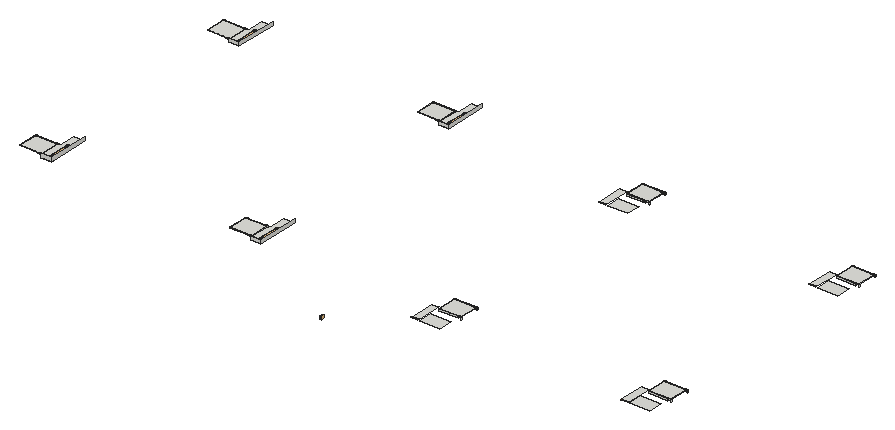
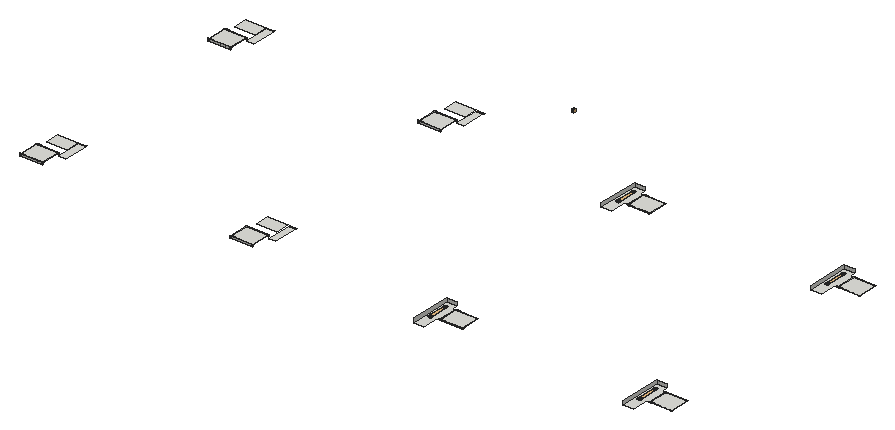
# SketchUp Ruby script. Lengths in inches.
U = 1.inch
M = Sketchup.active_model
def pt(a) = Geom::Point3d.new(a.map { |v| v * U })
def face(e, loops, mat)
  f = e.add_face(loops[0].map { |a| pt(a) })
  loops[1..].each { |l| e.add_face(l.map { |a| pt(a) }).erase! }
  f.material = f.back_material = mat if mat
  f
end
# faces: each face lists its corners as indices into pts; further lists are holes
def faces(e, pts, list, mat = nil) = list.each { |f| face(e, (f[0].is_a?(Array) ? f : [f]).map { |l| l.map { |i| pts[i] } }, mat) }
# xy, xz, yz: faces in a plane at the given z, y or x. An outline is a flat list of corners, or four numbers for a rectangle; further outlines are holes
def ring(l) = l.size == 4 ? [[l[0], l[1]], [l[2], l[1]], [l[2], l[3]], [l[0], l[3]]] : l.each_slice(2).to_a
def flat(e, list, mat, &to3) = list.each { |f| face(e, (f[0].is_a?(Array) ? f : [f]).map { |l| ring(l).map { |u, v| to3.(u, v) } }, mat) }
def xy(e, z, list, mat = nil) = flat(e, list, mat) { |x, y| [x, y, z] }
def xz(e, y, list, mat = nil) = flat(e, list, mat) { |x, z| [x, y, z] }
def yz(e, x, list, mat = nil) = flat(e, list, mat) { |y, z| [x, y, z] }
def lines(e, pts, list) = list.each { |a, b| e.add_line(pt(pts[a]), pt(pts[b])) }
# prism: a flat outline (further loops are holes) pulled along v
def prism(e, loops, v, mat = nil)
  f = face(e, loops, mat); d = Geom::Vector3d.new(v.map { |x| x * U })
  f.pushpull(f.normal.samedirection?(d) ? d.length : -d.length)
end
def box(e, o, s, mat = nil) = prism(e, [[o, [o[0] + s[0], o[1], o[2]], [o[0] + s[0], o[1] + s[1], o[2]], [o[0], o[1] + s[1], o[2]]]], [0, 0, s[2]], mat)
def at(x, y, z, deg = 0) = Geom::Transformation.translation(pt([x, y, z])) * Geom::Transformation.rotation(ORIGIN, Z_AXIS, deg.degrees)
def axes(o, x, y, z) = Geom::Transformation.new([*x, 0, *y, 0, *z, 0, *pt(o).to_a, 1])
def part(name) = M.definitions.add(name)
# library, detail: a bought-in or finely detailed component or shape, given as its bounding box
def library(name, o, s) = part(name).tap { |d| box(d.entities, o, s) }
def detail(e, o, s) = box(e.add_group.entities, o, s)
def put(e, d, t, mat = nil) = e.add_instance(d, t).tap { |i| i.material = mat if mat }
def group(e, t, mat = nil) = e.add_group.tap { |g| g.transformation = t; g.material = mat if mat }.entities
root = M.entities
M.materials.add("[Wood Veneer 01]").color = [76, 44, 23]
c1 = library("Spot Light",[-5.1,-5.1,-11.05],[10.2,10.2,11.05])
c2 = library("Group\#22",[-0.5,-0.5,-0.1],[13.19,93.55,0.2])
xy(root,93.875,[[2442.07,929.16,2442.76,929.47],[3334.66,929.16,3335.34,929.47],[2442.07,1928.52,2442.76,1928.83],[3334.66,1928.52,3335.34,1928.83]])
xy(root,97,[[563.18,847.15,656.89,931.09],[656.89,847.15,657.58,930.4],[1455.77,847.15,1549.48,931.09],[1549.48,847.15,1550.17,930.4],[563.18,931.09,645.68,931.22],
  [645.68,931.09,656.89,931.22],[1455.77,931.09,1538.27,931.22],[1538.27,931.09,1549.48,931.22],[563.18,1846.51,656.89,1930.45],[656.89,1846.51,657.58,1929.76],
  [1455.77,1846.51,1549.48,1930.45],[1549.48,1846.51,1550.17,1929.76],[563.18,1930.45,645.68,1930.57],[645.68,1930.45,656.89,1930.57],[1455.77,1930.45,1538.27,1930.57],
  [1538.27,1930.45,1549.48,1930.57]])
xy(root,97.25,[[656.89,847.15,657.58,930.4],[657.58,847.15,658.26,931.09],[1549.48,847.15,1550.17,930.4],[1550.17,847.15,1550.85,931.09],[656.89,930.4,657.58,931.09],
  [1549.48,930.4,1550.17,931.09],[656.89,931.09,657.58,931.47],[657.58,931.09,658.26,931.22],[1549.48,931.09,1550.17,931.47],[1550.17,931.09,1550.85,931.22],
  [656.89,1846.51,657.58,1929.76],[657.58,1846.51,658.26,1930.45],[1549.48,1846.51,1550.17,1929.76],[1550.17,1846.51,1550.85,1930.45],[656.89,1929.76,657.58,1930.45],
  [1549.48,1929.76,1550.17,1930.45],[656.89,1930.45,657.58,1930.82],[657.58,1930.45,658.26,1930.57],[1549.48,1930.45,1550.17,1930.82],[1550.17,1930.45,1550.85,1930.57]])
xy(root,97.9375,[[[671.36,824.85,671.36,847.15,662.14,847.15,662.14,931.78,671.36,931.78,671.36,1001.66,715.11,1001.66,715.11,824.85],[696.3,929.17,697.88,929.375,699.35,929.98,700.61,930.95,701.58,932.21,702.1875,933.68,702.39,935.26,702.1875,936.84,701.58,938.31,700.61,939.57,699.35,940.54,697.88,941.14,696.3,941.35,694.73,941.14,693.26,940.54,691.99,939.57,691.03,938.31,690.42,936.84,690.21,935.26,690.42,933.68,691.03,932.21,691.99,930.95,693.26,929.98,694.73,929.375],[696.3,848.8,697.85,849.01,699.3,849.6,700.54,850.56,701.5,851.8,702.1,853.25,702.3,854.8,702.1,856.35,701.5,857.8,700.54,859.04,699.3,860,697.85,860.6,696.3,860.8,694.75,860.6,693.3,860,692.06,859.04,691.11,857.8,690.51,856.35,690.3,854.8,690.51,853.25,691.11,851.8,692.06,850.56,693.3,849.6,694.75,849.01]],[[1563.95,824.85,1563.95,847.15,1554.73,847.15,1554.73,931.78,1563.95,931.78,1563.95,1001.66,1607.7,1001.66,1607.7,824.85],[1588.89,929.17,1590.47,929.375,1591.9375,929.98,1593.2,930.95,1594.17,932.21,1594.78,933.68,1594.98,935.26,1594.78,936.84,1594.17,938.31,1593.2,939.57,1591.9375,940.54,1590.47,941.14,1588.89,941.35,1587.31,941.14,1585.85,940.54,1584.58,939.57,1583.62,938.31,1583.01,936.84,1582.8,935.26,1583.01,933.68,1583.62,932.21,1584.58,930.95,1585.85,929.98,1587.31,929.375],[1588.89,848.8,1590.44,849.01,1591.89,849.6,1593.13,850.56,1594.09,851.8,1594.6875,853.25,1594.89,854.8,1594.6875,856.35,1594.09,857.8,1593.13,859.04,1591.89,860,1590.44,860.6,1588.89,860.8,1587.34,860.6,1585.89,860,1584.65,859.04,1583.7,857.8,1583.1,856.35,1582.89,854.8,1583.1,853.25,1583.7,851.8,1584.65,850.56,1585.89,849.6,1587.34,849.01]],[563.18,847.15,656.89,931.09],[656.89,847.15,657.58,931.78],[1455.77,847.15,1549.48,931.09],
  [1549.48,847.15,1550.17,931.78],[563.18,931.09,656.89,931.78],[657.58,931.09,658.26,931.09,658.26,931.22,662.14,931.22,662.14,931.78,657.58,931.78],[658.26,931.09,662.14,931.22],[1455.77,931.09,1549.48,931.78],
  [1550.17,931.09,1550.85,931.09,1550.85,931.22,1554.73,931.22,1554.73,931.78,1550.17,931.78],[1550.85,931.09,1554.73,931.22],[[671.36,1824.2,671.36,1846.51,662.14,1846.51,662.14,1931.13,671.36,1931.13,671.36,2001.02,715.11,2001.02,715.11,1824.2],[696.3,1928.52,697.88,1928.73,699.35,1929.34,700.61,1930.31,701.58,1931.57,702.1875,1933.04,702.39,1934.61,702.1875,1936.19,701.58,1937.66,700.61,1938.92,699.35,1939.89,697.88,1940.5,696.3,1940.71,694.73,1940.5,693.26,1939.89,691.99,1938.92,691.03,1937.66,690.42,1936.19,690.21,1934.61,690.42,1933.04,691.03,1931.57,691.99,1930.31,693.26,1929.34,694.73,1928.73],[696.3,1848.16,697.85,1848.36,699.3,1848.96,700.54,1849.91,701.5,1851.16,702.1,1852.6,702.3,1854.16,702.1,1855.71,701.5,1857.16,700.54,1858.4,699.3,1859.35,697.85,1859.95,696.3,1860.16,694.75,1859.95,693.3,1859.35,692.06,1858.4,691.11,1857.16,690.51,1855.71,690.3,1854.16,690.51,1852.6,691.11,1851.16,692.06,1849.91,693.3,1848.96,694.75,1848.36]],[[1563.95,1824.2,1563.95,1846.51,1554.73,1846.51,1554.73,1931.13,1563.95,1931.13,1563.95,2001.02,1607.7,2001.02,1607.7,1824.2],[1588.89,1928.52,1590.47,1928.73,1591.9375,1929.34,1593.2,1930.31,1594.17,1931.57,1594.78,1933.04,1594.98,1934.61,1594.78,1936.19,1594.17,1937.66,1593.2,1938.92,1591.9375,1939.89,1590.47,1940.5,1588.89,1940.71,1587.31,1940.5,1585.85,1939.89,1584.58,1938.92,1583.62,1937.66,1583.01,1936.19,1582.8,1934.61,1583.01,1933.04,1583.62,1931.57,1584.58,1930.31,1585.85,1929.34,1587.31,1928.73],[1588.89,1848.16,1590.44,1848.36,1591.89,1848.96,1593.13,1849.91,1594.09,1851.16,1594.6875,1852.6,1594.89,1854.16,1594.6875,1855.71,1594.09,1857.16,1593.13,1858.4,1591.89,1859.35,1590.44,1859.95,1588.89,1860.16,1587.34,1859.95,1585.89,1859.35,1584.65,1858.4,1583.7,1857.16,1583.1,1855.71,1582.89,1854.16,1583.1,1852.6,1583.7,1851.16,1584.65,1849.91,1585.89,1848.96,1587.34,1848.36]],[563.18,1846.51,656.89,1930.45],
  [656.89,1846.51,657.58,1931.13],[1455.77,1846.51,1549.48,1930.45],[1549.48,1846.51,1550.17,1931.13],[563.18,1930.45,656.89,1931.13],[657.58,1930.45,658.26,1930.45,658.26,1930.57,662.14,1930.57,662.14,1931.13,657.58,1931.13],
  [658.26,1930.45,662.14,1930.57],[1455.77,1930.45,1549.48,1931.13],[1550.17,1930.45,1550.85,1930.45,1550.85,1930.57,1554.73,1930.57,1554.73,1931.13,1550.17,1931.13],[1550.85,1930.45,1554.73,1930.57]])
xy(root,97.96,[[2346.59,747.5625,2430.86,806.0625],[3239.18,747.5625,3323.45,806.0625],[2346.59,1746.92,2430.86,1805.42],[3239.18,1746.92,3323.45,1805.42]])
xy(root,97.99,[[2308.36,747.5625,2338.14,753.47],[3200.95,747.5625,3230.73,753.47],[2308.36,1746.92,2338.14,1752.82],[3200.95,1746.92,3230.73,1752.82]],"[Wood Veneer 01]")
xy(root,101.6875,[[2348.36,844.85,2442.07,928.79],[2442.07,844.85,2442.76,928.1],[3240.94,844.85,3334.66,928.79],[3334.66,844.85,3335.34,928.1],[2348.36,928.79,2430.86,928.91],
  [2430.86,928.79,2442.07,928.91],[3240.94,928.79,3323.45,928.91],[3323.45,928.79,3334.66,928.91],[2348.36,1844.2,2442.07,1928.14],[2442.07,1844.2,2442.76,1927.45],
  [3240.94,1844.2,3334.66,1928.14],[3334.66,1844.2,3335.34,1927.45],[2348.36,1928.14,2430.86,1928.27],[2430.86,1928.14,2442.07,1928.27],[3240.94,1928.14,3323.45,1928.27],
  [3323.45,1928.14,3334.66,1928.27]])
xy(root,101.9375,[[2442.07,844.85,2442.76,928.1],[2442.76,844.85,2443.44,928.79],[3334.66,844.85,3335.34,928.1],[3335.34,844.85,3336.03,928.79],[2442.07,928.1,2442.76,928.79],
  [3334.66,928.1,3335.34,928.79],[2442.07,928.79,2442.76,929.16],[2442.76,928.79,2443.44,928.91],[3334.66,928.79,3335.34,929.16],[3335.34,928.79,3336.03,928.91],
  [2442.07,1844.2,2442.76,1927.45],[2442.76,1844.2,2443.44,1928.14],[3334.66,1844.2,3335.34,1927.45],[3335.34,1844.2,3336.03,1928.14],[2442.07,1927.45,2442.76,1928.14],
  [3334.66,1927.45,3335.34,1928.14],[2442.07,1928.14,2442.76,1928.52],[2442.76,1928.14,2443.44,1928.27],[3334.66,1928.14,3335.34,1928.52],[3335.34,1928.14,3336.03,1928.27]])
xz(root,824.85,[[671.36,97.9375,715.11,113.8125],[1563.95,97.9375,1607.7,113.8125]])
xz(root,844.85,[[2348.36,93.875,2430.86,101.6875],[2442.07,93.875,2442.76,101.6875],[2442.76,93.875,2447.32,93.875,2447.32,102.625,2443.44,102.625,2443.44,101.9375,2442.76,101.9375],[3240.94,93.875,3323.45,101.6875],[3334.66,93.875,3335.34,101.6875],
  [3335.34,93.875,3339.91,93.875,3339.91,102.625,3336.03,102.625,3336.03,101.9375,3335.34,101.9375],[2348.36,101.6875,2430.86,101.9375],[2430.86,101.6875,2442.07,101.9375],[2442.07,101.6875,2442.76,101.9375],[3240.94,101.6875,3323.45,101.9375],
  [3323.45,101.6875,3334.66,101.9375],[3334.66,101.6875,3335.34,101.9375],[2348.36,101.9375,2442.07,102.625],[2442.07,101.9375,2442.76,102.625],[2442.76,101.9375,2443.44,102.625],
  [3240.94,101.9375,3334.66,102.625],[3334.66,101.9375,3335.34,102.625],[3335.34,101.9375,3336.03,102.625]])
xz(root,847.15,[[563.18,97,645.68,97.25],[645.68,97,656.89,97.25],[656.89,97,657.58,97.25],[1455.77,97,1538.27,97.25],[1538.27,97,1549.48,97.25],
  [1549.48,97,1550.17,97.25],[563.18,97.25,656.89,97.9375],[656.89,97.25,657.58,97.9375],[657.58,97.25,658.26,97.9375],[1455.77,97.25,1549.48,97.9375],
  [1549.48,97.25,1550.17,97.9375],[1550.17,97.25,1550.85,97.9375]])
xz(root,928.1,[[2442.07,101.6875,2442.76,101.9375],[3334.66,101.6875,3335.34,101.9375]])
xz(root,928.79,[[2348.36,101.6875,2430.86,101.9375],[2430.86,101.6875,2442.07,101.9375],[3240.94,101.6875,3323.45,101.9375],[3323.45,101.6875,3334.66,101.9375],[2348.36,101.9375,2442.07,102.625],
  [2442.76,101.9375,2443.44,102.625],[3240.94,101.9375,3334.66,102.625],[3335.34,101.9375,3336.03,102.625]])
xz(root,929.16,[[2442.07,93.875,2442.76,101.9375],[3334.66,93.875,3335.34,101.9375]])
xz(root,929.47,[[2348.36,93.875,2442.07,102.625],[2442.07,93.875,2442.76,102.625],[2442.76,93.875,2447.32,102.625],[3240.94,93.875,3334.66,102.625],[3334.66,93.875,3335.34,102.625],
  [3335.34,93.875,3339.91,102.625]])
xz(root,930.4,[[656.89,97,657.58,97.25],[1549.48,97,1550.17,97.25]])
xz(root,931.09,[[563.18,97,645.68,97.25],[645.68,97,656.89,97.25],[1455.77,97,1538.27,97.25],[1538.27,97,1549.48,97.25],[563.18,97.25,656.89,97.9375],
  [657.58,97.25,658.26,97.9375],[1455.77,97.25,1549.48,97.9375],[1550.17,97.25,1550.85,97.9375]])
xz(root,1824.2,[[671.36,97.9375,715.11,113.8125],[1563.95,97.9375,1607.7,113.8125]])
xz(root,1844.2,[[2348.36,93.875,2430.86,101.6875],[2442.07,93.875,2442.76,101.6875],[2442.76,93.875,2447.32,93.875,2447.32,102.625,2443.44,102.625,2443.44,101.9375,2442.76,101.9375],[3240.94,93.875,3323.45,101.6875],[3334.66,93.875,3335.34,101.6875],
  [3335.34,93.875,3339.91,93.875,3339.91,102.625,3336.03,102.625,3336.03,101.9375,3335.34,101.9375],[2348.36,101.6875,2430.86,101.9375],[2430.86,101.6875,2442.07,101.9375],[2442.07,101.6875,2442.76,101.9375],[3240.94,101.6875,3323.45,101.9375],
  [3323.45,101.6875,3334.66,101.9375],[3334.66,101.6875,3335.34,101.9375],[2348.36,101.9375,2442.07,102.625],[2442.07,101.9375,2442.76,102.625],[2442.76,101.9375,2443.44,102.625],
  [3240.94,101.9375,3334.66,102.625],[3334.66,101.9375,3335.34,102.625],[3335.34,101.9375,3336.03,102.625]])
xz(root,1846.51,[[563.18,97,645.68,97.25],[645.68,97,656.89,97.25],[656.89,97,657.58,97.25],[1455.77,97,1538.27,97.25],[1538.27,97,1549.48,97.25],
  [1549.48,97,1550.17,97.25],[563.18,97.25,656.89,97.9375],[656.89,97.25,657.58,97.9375],[657.58,97.25,658.26,97.9375],[1455.77,97.25,1549.48,97.9375],
  [1549.48,97.25,1550.17,97.9375],[1550.17,97.25,1550.85,97.9375]])
xz(root,1927.45,[[2442.07,101.6875,2442.76,101.9375],[3334.66,101.6875,3335.34,101.9375]])
xz(root,1928.14,[[2348.36,101.6875,2430.86,101.9375],[2430.86,101.6875,2442.07,101.9375],[3240.94,101.6875,3323.45,101.9375],[3323.45,101.6875,3334.66,101.9375],[2348.36,101.9375,2442.07,102.625],
  [2442.76,101.9375,2443.44,102.625],[3240.94,101.9375,3334.66,102.625],[3335.34,101.9375,3336.03,102.625]])
xz(root,1928.52,[[2442.07,93.875,2442.76,101.9375],[3334.66,93.875,3335.34,101.9375]])
xz(root,1928.83,[[2348.36,93.875,2442.07,102.625],[2442.07,93.875,2442.76,102.625],[2442.76,93.875,2447.32,102.625],[3240.94,93.875,3334.66,102.625],[3334.66,93.875,3335.34,102.625],
  [3335.34,93.875,3339.91,102.625]])
xz(root,1929.76,[[656.89,97,657.58,97.25],[1549.48,97,1550.17,97.25]])
xz(root,1930.45,[[563.18,97,645.68,97.25],[645.68,97,656.89,97.25],[1455.77,97,1538.27,97.25],[1538.27,97,1549.48,97.25],[563.18,97.25,656.89,97.9375],
  [657.58,97.25,658.26,97.9375],[1455.77,97.25,1549.48,97.9375],[1550.17,97.25,1550.85,97.9375]])
yz(root,563.18,[[847.15,97,931.09,97.25],[1846.51,97,1930.45,97.25],[847.15,97.25,931.09,97.9375],[1846.51,97.25,1930.45,97.9375]])
yz(root,656.89,[[847.15,97,930.4,97.25],[930.4,97,931.09,97.25],[931.09,97,931.47,97.25],[1846.51,97,1929.76,97.25],[1929.76,97,1930.45,97.25],
  [1930.45,97,1930.82,97.25],[847.15,97.25,931.09,97.9375],[1846.51,97.25,1930.45,97.9375]])
yz(root,657.58,[[847.15,97,930.4,97.25],[1846.51,97,1929.76,97.25],[847.15,97.25,930.4,97.9375],[930.4,97.25,931.09,97.9375],[1846.51,97.25,1929.76,97.9375],
  [1929.76,97.25,1930.45,97.9375]])
yz(root,658.26,[[847.15,97.25,931.09,97.9375],[931.09,97.25,931.22,97.9375],[1846.51,97.25,1930.45,97.9375],[1930.45,97.25,1930.57,97.9375]])
yz(root,715.11,[[824.85,97.9375,1001.66,113.8125],[1824.2,97.9375,2001.02,113.8125]])
yz(root,1455.77,[[847.15,97,931.09,97.25],[1846.51,97,1930.45,97.25],[847.15,97.25,931.09,97.9375],[1846.51,97.25,1930.45,97.9375]])
yz(root,1549.48,[[847.15,97,930.4,97.25],[930.4,97,931.09,97.25],[931.09,97,931.47,97.25],[1846.51,97,1929.76,97.25],[1929.76,97,1930.45,97.25],
  [1930.45,97,1930.82,97.25],[847.15,97.25,931.09,97.9375],[1846.51,97.25,1930.45,97.9375]])
yz(root,1550.17,[[847.15,97,930.4,97.25],[1846.51,97,1929.76,97.25],[847.15,97.25,930.4,97.9375],[930.4,97.25,931.09,97.9375],[1846.51,97.25,1929.76,97.9375],
  [1929.76,97.25,1930.45,97.9375]])
yz(root,1550.85,[[847.15,97.25,931.09,97.9375],[931.09,97.25,931.22,97.9375],[1846.51,97.25,1930.45,97.9375],[1930.45,97.25,1930.57,97.9375]])
yz(root,1607.7,[[824.85,97.9375,1001.66,113.8125],[1824.2,97.9375,2001.02,113.8125]])
yz(root,2348.36,[[928.79,93.875,928.91,101.6875],[928.91,93.875,929.47,93.875,929.47,102.625,928.79,102.625,928.79,101.6875,928.91,101.6875],[1928.14,93.875,1928.27,101.6875],[1928.27,93.875,1928.83,93.875,1928.83,102.625,1928.14,102.625,1928.14,101.6875,1928.27,101.6875],[844.85,101.6875,928.79,101.9375],
  [1844.2,101.6875,1928.14,101.9375],[844.85,101.9375,928.79,102.625],[1844.2,101.9375,1928.14,102.625]])
yz(root,2442.07,[[929.16,93.875,929.16,101.9375,928.79,101.9375,928.79,102.625,929.47,102.625,929.47,93.875],[1928.52,93.875,1928.52,101.9375,1928.14,101.9375,1928.14,102.625,1928.83,102.625,1928.83,93.875],[844.85,101.6875,928.1,101.9375],[928.1,101.6875,928.79,101.9375],[928.79,101.6875,929.16,101.9375],
  [1844.2,101.6875,1927.45,101.9375],[1927.45,101.6875,1928.14,101.9375],[1928.14,101.6875,1928.52,101.9375],[844.85,101.9375,928.79,102.625],[1844.2,101.9375,1928.14,102.625]])
yz(root,2442.76,[[929.16,93.875,929.16,101.9375,928.79,101.9375,928.79,102.625,929.47,102.625,929.47,93.875],[928.91,93.875,929.16,101.9375],[1928.52,93.875,1928.52,101.9375,1928.14,101.9375,1928.14,102.625,1928.83,102.625,1928.83,93.875],[1928.27,93.875,1928.52,101.9375],[844.85,101.6875,928.1,101.9375],
  [1844.2,101.6875,1927.45,101.9375],[844.85,101.9375,928.1,102.625],[928.1,101.9375,928.79,102.625],[1844.2,101.9375,1927.45,102.625],[1927.45,101.9375,1928.14,102.625]])
yz(root,2443.44,[[844.85,101.9375,928.79,102.625],[928.79,101.9375,928.91,102.625],[1844.2,101.9375,1928.14,102.625],[1928.14,101.9375,1928.27,102.625]])
yz(root,2447.32,[[928.79,93.875,928.91,102.625],[928.91,93.875,929.47,102.625],[1928.14,93.875,1928.27,102.625],[1928.27,93.875,1928.83,102.625]])
yz(root,3240.94,[[928.79,93.875,928.91,101.6875],[928.91,93.875,929.47,93.875,929.47,102.625,928.79,102.625,928.79,101.6875,928.91,101.6875],[1928.14,93.875,1928.27,101.6875],[1928.27,93.875,1928.83,93.875,1928.83,102.625,1928.14,102.625,1928.14,101.6875,1928.27,101.6875],[844.85,101.6875,928.79,101.9375],
  [1844.2,101.6875,1928.14,101.9375],[844.85,101.9375,928.79,102.625],[1844.2,101.9375,1928.14,102.625]])
yz(root,3334.66,[[929.16,93.875,929.16,101.9375,928.79,101.9375,928.79,102.625,929.47,102.625,929.47,93.875],[1928.52,93.875,1928.52,101.9375,1928.14,101.9375,1928.14,102.625,1928.83,102.625,1928.83,93.875],[844.85,101.6875,928.1,101.9375],[928.1,101.6875,928.79,101.9375],[928.79,101.6875,929.16,101.9375],
  [1844.2,101.6875,1927.45,101.9375],[1927.45,101.6875,1928.14,101.9375],[1928.14,101.6875,1928.52,101.9375],[844.85,101.9375,928.79,102.625],[1844.2,101.9375,1928.14,102.625]])
yz(root,3335.34,[[929.16,93.875,929.16,101.9375,928.79,101.9375,928.79,102.625,929.47,102.625,929.47,93.875],[928.91,93.875,929.16,101.9375],[1928.52,93.875,1928.52,101.9375,1928.14,101.9375,1928.14,102.625,1928.83,102.625,1928.83,93.875],[1928.27,93.875,1928.52,101.9375],[844.85,101.6875,928.1,101.9375],
  [1844.2,101.6875,1927.45,101.9375],[844.85,101.9375,928.1,102.625],[928.1,101.9375,928.79,102.625],[1844.2,101.9375,1927.45,102.625],[1927.45,101.9375,1928.14,102.625]])
yz(root,3336.03,[[844.85,101.9375,928.79,102.625],[928.79,101.9375,928.91,102.625],[1844.2,101.9375,1928.14,102.625],[1928.14,101.9375,1928.27,102.625]])
yz(root,3339.91,[[928.79,93.875,928.91,102.625],[928.91,93.875,929.47,102.625],[1928.14,93.875,1928.27,102.625],[1928.27,93.875,1928.83,102.625]])
p = [[696.3,848.8,97.9375],[694.75,849.01,97.9375],[694.75,849.01,99.25],[696.3,848.8,99.25],[697.85,849.01,97.9375],[697.85,849.01,99.25],
  [1588.89,848.8,97.9375],[1587.34,849.01,97.9375],[1587.34,849.01,99.25],[1588.89,848.8,99.25],[1590.44,849.01,97.9375],[1590.44,849.01,99.25],
  [693.3,849.6,97.9375],[693.3,849.6,99.25],[699.3,849.6,97.9375],[699.3,849.6,99.25],[1585.89,849.6,97.9375],[1585.89,849.6,99.25],
  [1591.89,849.6,97.9375],[1591.89,849.6,99.25],[692.06,850.56,97.9375],[692.06,850.56,99.25],[700.54,850.56,97.9375],[700.54,850.56,99.25],
  [1584.65,850.56,97.9375],[1584.65,850.56,99.25],[1593.13,850.56,97.9375],[1593.13,850.56,99.25],[691.11,851.8,97.9375],[691.11,851.8,99.25],
  [701.5,851.8,97.9375],[701.5,851.8,99.25],[1583.7,851.8,97.9375],[1583.7,851.8,99.25],[1594.09,851.8,97.9375],[1594.09,851.8,99.25],
  [690.51,853.25,97.9375],[690.51,853.25,99.25],[702.1,853.25,97.9375],[702.1,853.25,99.25],[1583.1,853.25,97.9375],[1583.1,853.25,99.25],
  [1594.6875,853.25,97.9375],[1594.6875,853.25,99.25],[690.3,854.8,97.9375],[690.3,854.8,99.25],[702.3,854.8,97.9375],[702.3,854.8,99.25],
  [1582.89,854.8,97.9375],[1582.89,854.8,99.25],[1594.89,854.8,97.9375],[1594.89,854.8,99.25],[690.51,856.35,97.9375],[690.51,856.35,99.25],
  [702.1,856.35,97.9375],[702.1,856.35,99.25],[1583.1,856.35,97.9375],[1583.1,856.35,99.25],[1594.6875,856.35,97.9375],[1594.6875,856.35,99.25],
  [691.11,857.8,97.9375],[691.11,857.8,99.25],[701.5,857.8,97.9375],[701.5,857.8,99.25],[1583.7,857.8,97.9375],[1583.7,857.8,99.25],
  [1594.09,857.8,97.9375],[1594.09,857.8,99.25],[692.06,859.04,97.9375],[692.06,859.04,99.25],[700.54,859.04,97.9375],[700.54,859.04,99.25],
  [1584.65,859.04,97.9375],[1584.65,859.04,99.25],[1593.13,859.04,97.9375],[1593.13,859.04,99.25],[693.3,860,97.9375],[693.3,860,99.25],
  [699.3,860,97.9375],[699.3,860,99.25],[1585.89,860,97.9375],[1585.89,860,99.25],[1591.89,860,97.9375],[1591.89,860,99.25],
  [694.75,860.6,97.9375],[694.75,860.6,99.25],[697.85,860.6,97.9375],[697.85,860.6,99.25],[1587.34,860.6,97.9375],[1587.34,860.6,99.25],
  [1590.44,860.6,97.9375],[1590.44,860.6,99.25],[696.3,860.8,97.9375],[696.3,860.8,99.25],[1588.89,860.8,97.9375],[1588.89,860.8,99.25],
  [696.3,929.17,97.9375],[694.73,929.375,97.9375],[694.73,929.375,99.25],[696.3,929.17,99.25],[697.88,929.375,97.9375],[697.88,929.375,99.25],
  [1588.89,929.17,97.9375],[1587.31,929.375,97.9375],[1587.31,929.375,99.25],[1588.89,929.17,99.25],[1590.47,929.375,97.9375],[1590.47,929.375,99.25],
  [693.26,929.98,97.9375],[693.26,929.98,99.25],[699.35,929.98,97.9375],[699.35,929.98,99.25],[1585.85,929.98,97.9375],[1585.85,929.98,99.25],
  [1591.9375,929.98,97.9375],[1591.9375,929.98,99.25],[691.99,930.95,97.9375],[691.99,930.95,99.25],[700.61,930.95,97.9375],[700.61,930.95,99.25],
  [1584.58,930.95,97.9375],[1584.58,930.95,99.25],[1593.2,930.95,97.9375],[1593.2,930.95,99.25],[691.03,932.21,97.9375],[691.03,932.21,99.25],
  [701.58,932.21,97.9375],[701.58,932.21,99.25],[1583.62,932.21,97.9375],[1583.62,932.21,99.25],[1594.17,932.21,97.9375],[1594.17,932.21,99.25],
  [690.42,933.68,97.9375],[690.42,933.68,99.25],[702.1875,933.68,97.9375],[702.1875,933.68,99.25],[1583.01,933.68,97.9375],[1583.01,933.68,99.25],
  [1594.78,933.68,97.9375],[1594.78,933.68,99.25],[690.21,935.26,97.9375],[690.21,935.26,99.25],[702.39,935.26,97.9375],[702.39,935.26,99.25],
  [1582.8,935.26,97.9375],[1582.8,935.26,99.25],[1594.98,935.26,97.9375],[1594.98,935.26,99.25],[690.42,936.84,97.9375],[690.42,936.84,99.25],
  [702.1875,936.84,97.9375],[702.1875,936.84,99.25],[1583.01,936.84,97.9375],[1583.01,936.84,99.25],[1594.78,936.84,97.9375],[1594.78,936.84,99.25],
  [691.03,938.31,97.9375],[691.03,938.31,99.25],[701.58,938.31,97.9375],[701.58,938.31,99.25],[1583.62,938.31,97.9375],[1583.62,938.31,99.25],
  [1594.17,938.31,97.9375],[1594.17,938.31,99.25],[691.99,939.57,97.9375],[691.99,939.57,99.25],[700.61,939.57,97.9375],[700.61,939.57,99.25],
  [1584.58,939.57,97.9375],[1584.58,939.57,99.25],[1593.2,939.57,97.9375],[1593.2,939.57,99.25],[693.26,940.54,97.9375],[693.26,940.54,99.25],
  [699.35,940.54,97.9375],[699.35,940.54,99.25],[1585.85,940.54,97.9375],[1585.85,940.54,99.25],[1591.9375,940.54,97.9375],[1591.9375,940.54,99.25],
  [694.73,941.14,97.9375],[694.73,941.14,99.25],[697.88,941.14,97.9375],[697.88,941.14,99.25],[1587.31,941.14,97.9375],[1587.31,941.14,99.25],
  [1590.47,941.14,97.9375],[1590.47,941.14,99.25],[696.3,941.35,97.9375],[696.3,941.35,99.25],[1588.89,941.35,97.9375],[1588.89,941.35,99.25],
  [696.3,1848.16,97.9375],[694.75,1848.36,97.9375],[694.75,1848.36,99.25],[696.3,1848.16,99.25],[697.85,1848.36,97.9375],[697.85,1848.36,99.25],
  [1588.89,1848.16,97.9375],[1587.34,1848.36,97.9375],[1587.34,1848.36,99.25],[1588.89,1848.16,99.25],[1590.44,1848.36,97.9375],[1590.44,1848.36,99.25],
  [693.3,1848.96,97.9375],[693.3,1848.96,99.25],[699.3,1848.96,97.9375],[699.3,1848.96,99.25],[1585.89,1848.96,97.9375],[1585.89,1848.96,99.25],
  [1591.89,1848.96,97.9375],[1591.89,1848.96,99.25],[692.06,1849.91,97.9375],[692.06,1849.91,99.25],[700.54,1849.91,97.9375],[700.54,1849.91,99.25],
  [1584.65,1849.91,97.9375],[1584.65,1849.91,99.25],[1593.13,1849.91,97.9375],[1593.13,1849.91,99.25],[691.11,1851.16,97.9375],[691.11,1851.16,99.25],
  [701.5,1851.16,97.9375],[701.5,1851.16,99.25],[1583.7,1851.16,97.9375],[1583.7,1851.16,99.25],[1594.09,1851.16,97.9375],[1594.09,1851.16,99.25],
  [690.51,1852.6,97.9375],[690.51,1852.6,99.25],[702.1,1852.6,97.9375],[702.1,1852.6,99.25],[1583.1,1852.6,97.9375],[1583.1,1852.6,99.25],
  [1594.6875,1852.6,97.9375],[1594.6875,1852.6,99.25],[690.3,1854.16,97.9375],[690.3,1854.16,99.25],[702.3,1854.16,97.9375],[702.3,1854.16,99.25],
  [1582.89,1854.16,97.9375],[1582.89,1854.16,99.25],[1594.89,1854.16,97.9375],[1594.89,1854.16,99.25],[690.51,1855.71,97.9375],[690.51,1855.71,99.25],
  [702.1,1855.71,97.9375],[702.1,1855.71,99.25],[1583.1,1855.71,97.9375],[1583.1,1855.71,99.25],[1594.6875,1855.71,97.9375],[1594.6875,1855.71,99.25],
  [691.11,1857.16,97.9375],[691.11,1857.16,99.25],[701.5,1857.16,97.9375],[701.5,1857.16,99.25],[1583.7,1857.16,97.9375],[1583.7,1857.16,99.25],
  [1594.09,1857.16,97.9375],[1594.09,1857.16,99.25],[692.06,1858.4,97.9375],[692.06,1858.4,99.25],[700.54,1858.4,97.9375],[700.54,1858.4,99.25],
  [1584.65,1858.4,97.9375],[1584.65,1858.4,99.25],[1593.13,1858.4,97.9375],[1593.13,1858.4,99.25],[693.3,1859.35,97.9375],[693.3,1859.35,99.25],
  [699.3,1859.35,97.9375],[699.3,1859.35,99.25],[1585.89,1859.35,97.9375],[1585.89,1859.35,99.25],[1591.89,1859.35,97.9375],[1591.89,1859.35,99.25],
  [694.75,1859.95,97.9375],[694.75,1859.95,99.25],[697.85,1859.95,97.9375],[697.85,1859.95,99.25],[1587.34,1859.95,97.9375],[1587.34,1859.95,99.25],
  [1590.44,1859.95,97.9375],[1590.44,1859.95,99.25],[696.3,1860.16,97.9375],[696.3,1860.16,99.25],[1588.89,1860.16,97.9375],[1588.89,1860.16,99.25],
  [696.3,1928.52,97.9375],[694.73,1928.73,97.9375],[694.73,1928.73,99.25],[696.3,1928.52,99.25],[697.88,1928.73,97.9375],[697.88,1928.73,99.25],
  [1588.89,1928.52,97.9375],[1587.31,1928.73,97.9375],[1587.31,1928.73,99.25],[1588.89,1928.52,99.25],[1590.47,1928.73,97.9375],[1590.47,1928.73,99.25],
  [693.26,1929.34,97.9375],[693.26,1929.34,99.25],[699.35,1929.34,97.9375],[699.35,1929.34,99.25],[1585.85,1929.34,97.9375],[1585.85,1929.34,99.25],
  [1591.9375,1929.34,97.9375],[1591.9375,1929.34,99.25],[691.99,1930.31,97.9375],[691.99,1930.31,99.25],[700.61,1930.31,97.9375],[700.61,1930.31,99.25],
  [1584.58,1930.31,97.9375],[1584.58,1930.31,99.25],[1593.2,1930.31,97.9375],[1593.2,1930.31,99.25],[691.03,1931.57,97.9375],[691.03,1931.57,99.25],
  [701.58,1931.57,97.9375],[701.58,1931.57,99.25],[1583.62,1931.57,97.9375],[1583.62,1931.57,99.25],[1594.17,1931.57,97.9375],[1594.17,1931.57,99.25],
  [690.42,1933.04,97.9375],[690.42,1933.04,99.25],[702.1875,1933.04,97.9375],[702.1875,1933.04,99.25],[1583.01,1933.04,97.9375],[1583.01,1933.04,99.25],
  [1594.78,1933.04,97.9375],[1594.78,1933.04,99.25],[690.21,1934.61,97.9375],[690.21,1934.61,99.25],[702.39,1934.61,97.9375],[702.39,1934.61,99.25],
  [1582.8,1934.61,97.9375],[1582.8,1934.61,99.25],[1594.98,1934.61,97.9375],[1594.98,1934.61,99.25],[690.42,1936.19,97.9375],[690.42,1936.19,99.25],
  [702.1875,1936.19,97.9375],[702.1875,1936.19,99.25],[1583.01,1936.19,97.9375],[1583.01,1936.19,99.25],[1594.78,1936.19,97.9375],[1594.78,1936.19,99.25],
  [691.03,1937.66,97.9375],[691.03,1937.66,99.25],[701.58,1937.66,97.9375],[701.58,1937.66,99.25],[1583.62,1937.66,97.9375],[1583.62,1937.66,99.25],
  [1594.17,1937.66,97.9375],[1594.17,1937.66,99.25],[691.99,1938.92,97.9375],[691.99,1938.92,99.25],[700.61,1938.92,97.9375],[700.61,1938.92,99.25],
  [1584.58,1938.92,97.9375],[1584.58,1938.92,99.25],[1593.2,1938.92,97.9375],[1593.2,1938.92,99.25],[693.26,1939.89,97.9375],[693.26,1939.89,99.25],
  [699.35,1939.89,97.9375],[699.35,1939.89,99.25],[1585.85,1939.89,97.9375],[1585.85,1939.89,99.25],[1591.9375,1939.89,97.9375],[1591.9375,1939.89,99.25],
  [694.73,1940.5,97.9375],[694.73,1940.5,99.25],[697.88,1940.5,97.9375],[697.88,1940.5,99.25],[1587.31,1940.5,97.9375],[1587.31,1940.5,99.25],
  [1590.47,1940.5,97.9375],[1590.47,1940.5,99.25],[696.3,1940.71,97.9375],[696.3,1940.71,99.25],[1588.89,1940.71,97.9375],[1588.89,1940.71,99.25],
  [2307.7,857.25,97.96],[2338.14,857.25,97.96],[2338.14,753.47,97.99],[2308.36,753.47,97.99],[3200.29,857.25,97.96],[3230.73,857.25,97.96],
  [3230.73,753.47,97.99],[3200.95,753.47,97.99],[2307.7,1856.6,97.96],[2338.14,1856.6,97.96],[2338.14,1752.82,97.99],[2308.36,1752.82,97.99],
  [3200.29,1856.6,97.96],[3230.73,1856.6,97.96],[3230.73,1752.82,97.99],[3200.95,1752.82,97.99],[2305.34,753.47,100.32],[2305.34,747.5625,100.32],
  [3197.93,753.47,100.32],[3197.93,747.5625,100.32],[520.16,755.77,95.64],[520.16,749.87,95.64],[1412.75,755.77,95.64],[1412.75,749.87,95.64],
  [2305.34,1752.82,100.32],[2305.34,1746.92,100.32],[3197.93,1752.82,100.32],[3197.93,1746.92,100.32],[520.16,1755.13,95.64],[520.16,1749.22,95.64],
  [1412.75,1755.13,95.64],[1412.75,1749.22,95.64]]
faces(root,p,[[0,1,2,3],[4,0,3,5],[6,7,8,9],[10,6,9,11],[1,12,13,2],[14,4,5,15],[7,16,17,8],[18,10,11,19],
  [12,20,21,13],[22,14,15,23],[16,24,25,17],[26,18,19,27],[20,28,29,21],[30,22,23,31],[24,32,33,25],[34,26,27,35],
  [28,36,37,29],[38,30,31,39],[32,40,41,33],[42,34,35,43],[36,44,45,37],[46,38,39,47],[40,48,49,41],[50,42,43,51],
  [44,52,53,45],[54,46,47,55],[48,56,57,49],[58,50,51,59],[52,60,61,53],[62,54,55,63],[56,64,65,57],[66,58,59,67],
  [60,68,69,61],[70,62,63,71],[64,72,73,65],[74,66,67,75],[68,76,77,69],[78,70,71,79],[72,80,81,73],[82,74,75,83],
  [76,84,85,77],[86,78,79,87],[80,88,89,81],[90,82,83,91],[84,92,93,85],[92,86,87,93],[88,94,95,89],[94,90,91,95],
  [96,97,98,99],[100,96,99,101],[102,103,104,105],[106,102,105,107],[97,108,109,98],[110,100,101,111],[103,112,113,104],[114,106,107,115],
  [108,116,117,109],[118,110,111,119],[112,120,121,113],[122,114,115,123],[116,124,125,117],[126,118,119,127],[120,128,129,121],[130,122,123,131],
  [124,132,133,125],[134,126,127,135],[128,136,137,129],[138,130,131,139],[132,140,141,133],[142,134,135,143],[136,144,145,137],[146,138,139,147],
  [140,148,149,141],[150,142,143,151],[144,152,153,145],[154,146,147,155],[148,156,157,149],[158,150,151,159],[152,160,161,153],[162,154,155,163],
  [156,164,165,157],[166,158,159,167],[160,168,169,161],[170,162,163,171],[164,172,173,165],[174,166,167,175],[168,176,177,169],[178,170,171,179],
  [172,180,181,173],[182,174,175,183],[176,184,185,177],[186,178,179,187],[180,188,189,181],[188,182,183,189],[184,190,191,185],[190,186,187,191],
  [192,193,194,195],[196,192,195,197],[198,199,200,201],[202,198,201,203],[193,204,205,194],[206,196,197,207],[199,208,209,200],[210,202,203,211],
  [204,212,213,205],[214,206,207,215],[208,216,217,209],[218,210,211,219],[212,220,221,213],[222,214,215,223],[216,224,225,217],[226,218,219,227],
  [220,228,229,221],[230,222,223,231],[224,232,233,225],[234,226,227,235],[228,236,237,229],[238,230,231,239],[232,240,241,233],[242,234,235,243],
  [236,244,245,237],[246,238,239,247],[240,248,249,241],[250,242,243,251],[244,252,253,245],[254,246,247,255],[248,256,257,249],[258,250,251,259],
  [252,260,261,253],[262,254,255,263],[256,264,265,257],[266,258,259,267],[260,268,269,261],[270,262,263,271],[264,272,273,265],[274,266,267,275],
  [268,276,277,269],[278,270,271,279],[272,280,281,273],[282,274,275,283],[276,284,285,277],[284,278,279,285],[280,286,287,281],[286,282,283,287],
  [288,289,290,291],[292,288,291,293],[294,295,296,297],[298,294,297,299],[289,300,301,290],[302,292,293,303],[295,304,305,296],[306,298,299,307],
  [300,308,309,301],[310,302,303,311],[304,312,313,305],[314,306,307,315],[308,316,317,309],[318,310,311,319],[312,320,321,313],[322,314,315,323],
  [316,324,325,317],[326,318,319,327],[320,328,329,321],[330,322,323,331],[324,332,333,325],[334,326,327,335],[328,336,337,329],[338,330,331,339],
  [332,340,341,333],[342,334,335,343],[336,344,345,337],[346,338,339,347],[340,348,349,341],[350,342,343,351],[344,352,353,345],[354,346,347,355],
  [348,356,357,349],[358,350,351,359],[352,360,361,353],[362,354,355,363],[356,364,365,357],[366,358,359,367],[360,368,369,361],[370,362,363,371],
  [364,372,373,365],[374,366,367,375],[368,376,377,369],[378,370,371,379],[372,380,381,373],[380,374,375,381],[376,382,383,377],[382,378,379,383],
  [384,385,386,387],[388,389,390,391],[392,393,394,395],[396,397,398,399]])
lines(root,p,[[400,401],[402,403],[404,405],[406,407],[408,409],[410,411],[412,413],[414,415]])
put(root,c1,at(2081.51,554.38,109.62))
put(root,c2,at(690.21,1848.16,99.25))
put(root,c2,at(690.21,848.8,99.25))
put(root,c2,at(1582.8,1848.16,99.25))
put(root,c2,at(1582.8,848.8,99.25))
